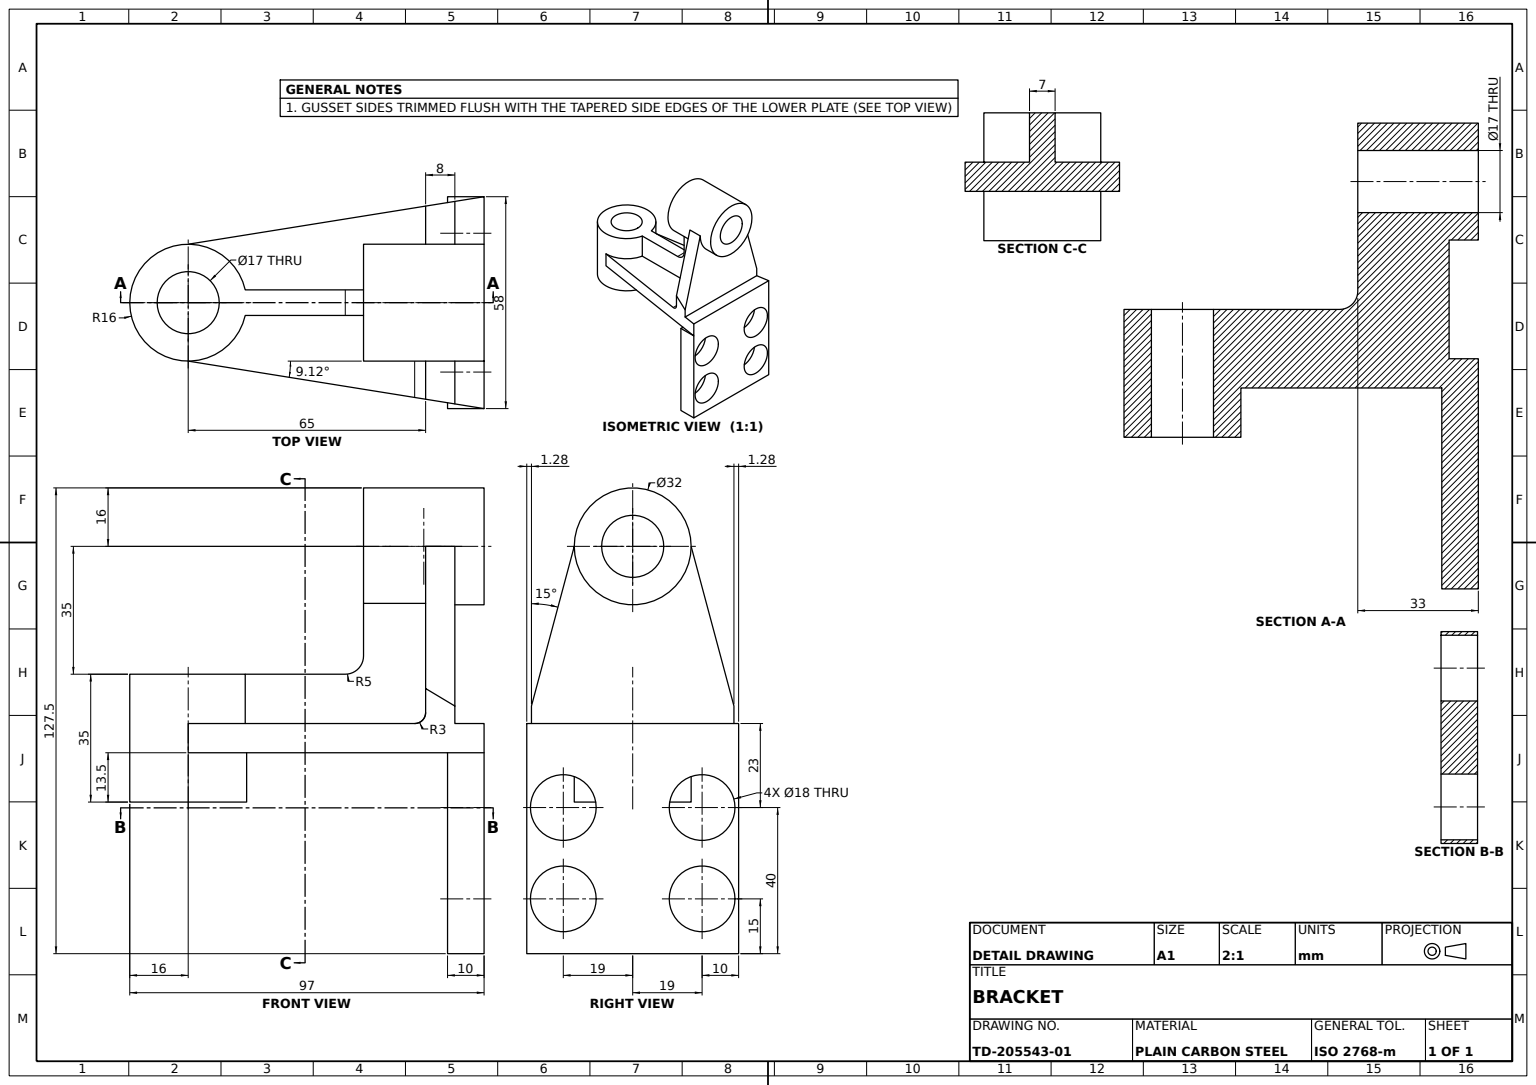
ISO-10303-21;
HEADER;
FILE_DESCRIPTION((''),'2;1');
FILE_NAME('','',(''),(''),'','','');
FILE_SCHEMA(('AUTOMOTIVE_DESIGN'));
ENDSEC;
DATA;
#1=APPLICATION_CONTEXT('');
#2=PRODUCT_CONTEXT('',#1,'mechanical');
#3=PRODUCT('','','',(#2));
#4=PRODUCT_DEFINITION_FORMATION('','',#3);
#5=PRODUCT_DEFINITION_CONTEXT('',#1,'design');
#6=PRODUCT_DEFINITION('','',#4,#5);
#7=PRODUCT_DEFINITION_SHAPE('','',#6);
#8=(LENGTH_UNIT()NAMED_UNIT(*)SI_UNIT(.MILLI.,.METRE.));
#9=(NAMED_UNIT(*)PLANE_ANGLE_UNIT()SI_UNIT($,.RADIAN.));
#10=(NAMED_UNIT(*)SI_UNIT($,.STERADIAN.)SOLID_ANGLE_UNIT());
#11=UNCERTAINTY_MEASURE_WITH_UNIT(LENGTH_MEASURE(1.E-05),#8,'distance_accuracy_value','');
#12=(GEOMETRIC_REPRESENTATION_CONTEXT(3)GLOBAL_UNCERTAINTY_ASSIGNED_CONTEXT((#11))GLOBAL_UNIT_ASSIGNED_CONTEXT((#8,#9,#10))REPRESENTATION_CONTEXT('',''));
#13=CARTESIAN_POINT('',(26.432099,13.580247,-65.));
#14=VERTEX_POINT('',#13);
#15=CARTESIAN_POINT('',(26.432099,7.,-65.));
#16=VERTEX_POINT('',#15);
#17=CARTESIAN_POINT('',(26.432099,52.5,-65.));
#18=DIRECTION('',(0.,-1.,0.));
#19=VECTOR('',#18,1000.);
#20=LINE('',#17,#19);
#21=EDGE_CURVE('',#14,#16,#20,.T.);
#22=ORIENTED_EDGE('',*,*,#21,.F.);
#23=CARTESIAN_POINT('',(16.,52.5,-65.));
#24=VERTEX_POINT('',#23);
#25=DIRECTION('',(-0.258901995,0.965903596,0.));
#26=VECTOR('',#25,1000.);
#27=LINE('',#23,#26);
#28=EDGE_CURVE('',#14,#24,#27,.T.);
#29=ORIENTED_EDGE('',*,*,#28,.T.);
#30=CARTESIAN_POINT('',(3.5,36.887505,-65.));
#31=VERTEX_POINT('',#30);
#32=CARTESIAN_POINT('',(0.,52.5,-65.));
#33=DIRECTION('',(0.,0.,-1.));
#34=DIRECTION('',(1.,0.,0.));
#35=AXIS2_PLACEMENT_3D('',#32,#33,#34);
#36=CIRCLE('',#35,16.);
#37=EDGE_CURVE('',#24,#31,#36,.T.);
#38=ORIENTED_EDGE('',*,*,#37,.T.);
#39=CARTESIAN_POINT('',(3.5,7.,-65.));
#40=VERTEX_POINT('',#39);
#41=CARTESIAN_POINT('',(3.5,4.,-65.));
#42=DIRECTION('',(0.,1.,0.));
#43=VECTOR('',#42,1000.);
#44=LINE('',#41,#43);
#45=EDGE_CURVE('',#40,#31,#44,.T.);
#46=ORIENTED_EDGE('',*,*,#45,.F.);
#47=VECTOR('',#34,1000.);
#48=LINE('',#15,#47);
#49=EDGE_CURVE('',#40,#16,#48,.T.);
#50=ORIENTED_EDGE('',*,*,#49,.T.);
#51=EDGE_LOOP('',(#22,#29,#38,#46,#50));
#52=FACE_OUTER_BOUND('',#51,.T.);
#53=DIRECTION('',(0.,0.,1.));
#54=AXIS2_PLACEMENT_3D('',#32,#53,#34);
#55=PLANE('',#54);
#56=ADVANCED_FACE('',(#52),#55,.T.);
#57=CARTESIAN_POINT('',(28.,-44.,-71.));
#58=VERTEX_POINT('',#57);
#59=CARTESIAN_POINT('',(10.,-44.,-71.));
#60=VERTEX_POINT('',#59);
#61=CARTESIAN_POINT('',(19.,-44.,-71.));
#62=AXIS2_PLACEMENT_3D('',#61,#53,#34);
#63=CIRCLE('',#62,9.);
#64=EDGE_CURVE('',#58,#60,#63,.T.);
#65=ORIENTED_EDGE('',*,*,#64,.T.);
#66=CARTESIAN_POINT('',(10.,-44.,-81.));
#67=VERTEX_POINT('',#66);
#68=CARTESIAN_POINT('',(10.,-44.,-126.));
#69=VECTOR('',#53,1000.);
#70=LINE('',#68,#69);
#71=EDGE_CURVE('',#67,#60,#70,.T.);
#72=ORIENTED_EDGE('',*,*,#71,.F.);
#73=CARTESIAN_POINT('',(28.,-44.,-81.));
#74=VERTEX_POINT('',#73);
#75=CARTESIAN_POINT('',(19.,-44.,-81.));
#76=AXIS2_PLACEMENT_3D('',#75,#53,#34);
#77=CIRCLE('',#76,9.);
#78=EDGE_CURVE('',#74,#67,#77,.T.);
#79=ORIENTED_EDGE('',*,*,#78,.F.);
#80=CARTESIAN_POINT('',(28.,-44.,-126.));
#81=LINE('',#80,#69);
#82=EDGE_CURVE('',#74,#58,#81,.T.);
#83=ORIENTED_EDGE('',*,*,#82,.T.);
#84=EDGE_LOOP('',(#65,#72,#79,#83));
#85=FACE_OUTER_BOUND('',#84,.T.);
#86=CARTESIAN_POINT('',(19.,-44.,-126.));
#87=AXIS2_PLACEMENT_3D('',#86,#53,#34);
#88=CYLINDRICAL_SURFACE('',#87,9.);
#89=ADVANCED_FACE('',(#85),#88,.F.);
#90=CARTESIAN_POINT('',(-28.,-44.,-81.));
#91=VERTEX_POINT('',#90);
#92=CARTESIAN_POINT('',(-28.,-44.,-71.));
#93=VERTEX_POINT('',#92);
#94=CARTESIAN_POINT('',(-28.,-44.,-126.));
#95=LINE('',#94,#69);
#96=EDGE_CURVE('',#91,#93,#95,.T.);
#97=ORIENTED_EDGE('',*,*,#96,.F.);
#98=CARTESIAN_POINT('',(-10.,-44.,-81.));
#99=VERTEX_POINT('',#98);
#100=CARTESIAN_POINT('',(-19.,-44.,-81.));
#101=AXIS2_PLACEMENT_3D('',#100,#53,#34);
#102=CIRCLE('',#101,9.);
#103=EDGE_CURVE('',#99,#91,#102,.T.);
#104=ORIENTED_EDGE('',*,*,#103,.F.);
#105=CARTESIAN_POINT('',(-10.,-44.,-71.));
#106=VERTEX_POINT('',#105);
#107=CARTESIAN_POINT('',(-10.,-44.,-126.));
#108=LINE('',#107,#69);
#109=EDGE_CURVE('',#99,#106,#108,.T.);
#110=ORIENTED_EDGE('',*,*,#109,.T.);
#111=CARTESIAN_POINT('',(-19.,-44.,-71.));
#112=DIRECTION('',(-1.,0.,0.));
#113=AXIS2_PLACEMENT_3D('',#111,#53,#112);
#114=CIRCLE('',#113,9.);
#115=EDGE_CURVE('',#106,#93,#114,.T.);
#116=ORIENTED_EDGE('',*,*,#115,.T.);
#117=EDGE_LOOP('',(#97,#104,#110,#116));
#118=FACE_OUTER_BOUND('',#117,.T.);
#119=CARTESIAN_POINT('',(-19.,-44.,-126.));
#120=AXIS2_PLACEMENT_3D('',#119,#53,#34);
#121=CYLINDRICAL_SURFACE('',#120,9.);
#122=ADVANCED_FACE('',(#118),#121,.F.);
#123=CARTESIAN_POINT('',(-16.,52.5,-73.));
#124=VERTEX_POINT('',#123);
#125=CARTESIAN_POINT('',(-27.716049,8.790123,-73.));
#126=VERTEX_POINT('',#125);
#127=DIRECTION('',(-0.258901995,-0.965903596,0.));
#128=VECTOR('',#127,1000.);
#129=LINE('',#123,#128);
#130=EDGE_CURVE('',#124,#126,#129,.T.);
#131=ORIENTED_EDGE('',*,*,#130,.T.);
#132=CARTESIAN_POINT('',(-26.432099,13.580247,-65.));
#133=VERTEX_POINT('',#132);
#134=CARTESIAN_POINT('',(-24.463652,20.924069,-52.73506));
#135=DIRECTION('',(-0.136410131,-0.50891472,-0.849940047));
#136=VECTOR('',#135,1000.);
#137=LINE('',#134,#136);
#138=EDGE_CURVE('',#133,#126,#137,.T.);
#139=ORIENTED_EDGE('',*,*,#138,.F.);
#140=CARTESIAN_POINT('',(-16.,52.5,-65.));
#141=VERTEX_POINT('',#140);
#142=LINE('',#140,#128);
#143=EDGE_CURVE('',#141,#133,#142,.T.);
#144=ORIENTED_EDGE('',*,*,#143,.F.);
#145=LINE('',#123,#69);
#146=EDGE_CURVE('',#124,#141,#145,.T.);
#147=ORIENTED_EDGE('',*,*,#146,.F.);
#148=EDGE_LOOP('',(#131,#139,#144,#147));
#149=FACE_OUTER_BOUND('',#148,.T.);
#150=DIRECTION('',(-0.965903596,0.258901995,0.));
#151=AXIS2_PLACEMENT_3D('',#123,#150,#127);
#152=PLANE('',#151);
#153=ADVANCED_FACE('',(#149),#152,.T.);
#154=CARTESIAN_POINT('',(-29.,-4.,-71.));
#155=VERTEX_POINT('',#154);
#156=CARTESIAN_POINT('',(-29.,-4.,-81.));
#157=VERTEX_POINT('',#156);
#158=VECTOR('',#33,1000.);
#159=LINE('',#154,#158);
#160=EDGE_CURVE('',#155,#157,#159,.T.);
#161=ORIENTED_EDGE('',*,*,#160,.F.);
#162=CARTESIAN_POINT('',(-27.395062,-4.,-71.));
#163=VERTEX_POINT('',#162);
#164=CARTESIAN_POINT('',(29.,-4.,-71.));
#165=VECTOR('',#112,1000.);
#166=LINE('',#164,#165);
#167=EDGE_CURVE('',#163,#155,#166,.T.);
#168=ORIENTED_EDGE('',*,*,#167,.F.);
#169=DIRECTION('',(0.1584659,0.,0.987364451));
#170=VECTOR('',#169,1000.);
#171=LINE('',#156,#170);
#172=EDGE_CURVE('',#157,#163,#171,.T.);
#173=ORIENTED_EDGE('',*,*,#172,.F.);
#174=EDGE_LOOP('',(#161,#168,#173));
#175=FACE_OUTER_BOUND('',#174,.T.);
#176=CARTESIAN_POINT('',(0.,-4.,0.));
#177=AXIS2_PLACEMENT_3D('',#176,#18,#33);
#178=PLANE('',#177);
#179=ADVANCED_FACE('',(#175),#178,.F.);
#180=CARTESIAN_POINT('',(0.,-17.5,8.5));
#181=VERTEX_POINT('',#180);
#182=CARTESIAN_POINT('',(0.,17.5,8.5));
#183=VERTEX_POINT('',#182);
#184=CARTESIAN_POINT('',(0.,-39.5,8.5));
#185=LINE('',#184,#43);
#186=EDGE_CURVE('',#181,#183,#185,.T.);
#187=ORIENTED_EDGE('',*,*,#186,.T.);
#188=CARTESIAN_POINT('',(0.,17.5,-8.5));
#189=VERTEX_POINT('',#188);
#190=CARTESIAN_POINT('',(0.,17.5,0.));
#191=AXIS2_PLACEMENT_3D('',#190,#42,#53);
#192=CIRCLE('',#191,8.5);
#193=EDGE_CURVE('',#183,#189,#192,.T.);
#194=ORIENTED_EDGE('',*,*,#193,.T.);
#195=CARTESIAN_POINT('',(0.,-17.5,-8.5));
#196=VERTEX_POINT('',#195);
#197=CARTESIAN_POINT('',(0.,-39.5,-8.5));
#198=LINE('',#197,#43);
#199=EDGE_CURVE('',#196,#189,#198,.T.);
#200=ORIENTED_EDGE('',*,*,#199,.F.);
#201=CARTESIAN_POINT('',(0.,-17.5,0.));
#202=AXIS2_PLACEMENT_3D('',#201,#42,#53);
#203=CIRCLE('',#202,8.5);
#204=EDGE_CURVE('',#181,#196,#203,.T.);
#205=ORIENTED_EDGE('',*,*,#204,.F.);
#206=EDGE_LOOP('',(#187,#194,#200,#205));
#207=FACE_OUTER_BOUND('',#206,.T.);
#208=CARTESIAN_POINT('',(0.,-39.5,0.));
#209=AXIS2_PLACEMENT_3D('',#208,#42,#53);
#210=CYLINDRICAL_SURFACE('',#209,8.5);
#211=ADVANCED_FACE('',(#207),#210,.F.);
#212=VERTEX_POINT('',#164);
#213=CARTESIAN_POINT('',(27.395062,-4.,-71.));
#214=VERTEX_POINT('',#213);
#215=EDGE_CURVE('',#212,#214,#166,.T.);
#216=ORIENTED_EDGE('',*,*,#215,.F.);
#217=CARTESIAN_POINT('',(29.,-4.,-81.));
#218=VERTEX_POINT('',#217);
#219=LINE('',#217,#69);
#220=EDGE_CURVE('',#218,#212,#219,.T.);
#221=ORIENTED_EDGE('',*,*,#220,.F.);
#222=DIRECTION('',(0.1584659,0.,-0.987364451));
#223=VECTOR('',#222,1000.);
#224=LINE('',#217,#223);
#225=EDGE_CURVE('',#214,#218,#224,.T.);
#226=ORIENTED_EDGE('',*,*,#225,.F.);
#227=EDGE_LOOP('',(#216,#221,#226));
#228=FACE_OUTER_BOUND('',#227,.T.);
#229=ADVANCED_FACE('',(#228),#178,.F.);
#230=ORIENTED_EDGE('',*,*,#199,.T.);
#231=EDGE_CURVE('',#189,#183,#192,.T.);
#232=ORIENTED_EDGE('',*,*,#231,.T.);
#233=ORIENTED_EDGE('',*,*,#186,.F.);
#234=EDGE_CURVE('',#196,#181,#203,.T.);
#235=ORIENTED_EDGE('',*,*,#234,.F.);
#236=EDGE_LOOP('',(#230,#232,#233,#235));
#237=FACE_OUTER_BOUND('',#236,.T.);
#238=ADVANCED_FACE('',(#237),#210,.F.);
#239=CARTESIAN_POINT('',(-29.,4.,-81.));
#240=VERTEX_POINT('',#239);
#241=CARTESIAN_POINT('',(-27.716049,4.,-73.));
#242=VERTEX_POINT('',#241);
#243=LINE('',#239,#170);
#244=EDGE_CURVE('',#240,#242,#243,.T.);
#245=ORIENTED_EDGE('',*,*,#244,.T.);
#246=CARTESIAN_POINT('',(27.716049,4.,-73.));
#247=VERTEX_POINT('',#246);
#248=CARTESIAN_POINT('',(0.,4.,-73.));
#249=LINE('',#248,#47);
#250=EDGE_CURVE('',#242,#247,#249,.T.);
#251=ORIENTED_EDGE('',*,*,#250,.T.);
#252=CARTESIAN_POINT('',(29.,4.,-81.));
#253=VERTEX_POINT('',#252);
#254=LINE('',#252,#223);
#255=EDGE_CURVE('',#247,#253,#254,.T.);
#256=ORIENTED_EDGE('',*,*,#255,.T.);
#257=CARTESIAN_POINT('',(0.,4.,-81.));
#258=LINE('',#257,#165);
#259=EDGE_CURVE('',#253,#240,#258,.T.);
#260=ORIENTED_EDGE('',*,*,#259,.T.);
#261=EDGE_LOOP('',(#245,#251,#256,#260));
#262=FACE_OUTER_BOUND('',#261,.T.);
#263=CARTESIAN_POINT('',(0.,4.,0.));
#264=AXIS2_PLACEMENT_3D('',#263,#42,#53);
#265=PLANE('',#264);
#266=ADVANCED_FACE('',(#262),#265,.T.);
#267=CARTESIAN_POINT('',(0.,-17.5,16.));
#268=VERTEX_POINT('',#267);
#269=CARTESIAN_POINT('',(0.,-17.5,-16.));
#270=VERTEX_POINT('',#269);
#271=CIRCLE('',#202,16.);
#272=EDGE_CURVE('',#268,#270,#271,.T.);
#273=ORIENTED_EDGE('',*,*,#272,.F.);
#274=EDGE_CURVE('',#270,#268,#271,.T.);
#275=ORIENTED_EDGE('',*,*,#274,.F.);
#276=EDGE_LOOP('',(#273,#275));
#277=FACE_OUTER_BOUND('',#276,.T.);
#278=ORIENTED_EDGE('',*,*,#234,.T.);
#279=ORIENTED_EDGE('',*,*,#204,.T.);
#280=EDGE_LOOP('',(#278,#279));
#281=FACE_BOUND('',#280,.T.);
#282=PLANE('',#202);
#283=ADVANCED_FACE('',(#277,#281),#282,.F.);
#284=CARTESIAN_POINT('',(-26.432099,4.,-65.));
#285=VERTEX_POINT('',#284);
#286=CARTESIAN_POINT('',(-16.,4.,0.));
#287=VERTEX_POINT('',#286);
#288=EDGE_CURVE('',#285,#287,#243,.T.);
#289=ORIENTED_EDGE('',*,*,#288,.F.);
#290=CARTESIAN_POINT('',(-26.432099,52.5,-65.));
#291=LINE('',#290,#43);
#292=EDGE_CURVE('',#285,#133,#291,.T.);
#293=ORIENTED_EDGE('',*,*,#292,.T.);
#294=ORIENTED_EDGE('',*,*,#138,.T.);
#295=CARTESIAN_POINT('',(-27.716049,34.,-73.));
#296=LINE('',#295,#19);
#297=EDGE_CURVE('',#126,#242,#296,.T.);
#298=ORIENTED_EDGE('',*,*,#297,.T.);
#299=ORIENTED_EDGE('',*,*,#244,.F.);
#300=LINE('',#239,#19);
#301=EDGE_CURVE('',#240,#157,#300,.T.);
#302=ORIENTED_EDGE('',*,*,#301,.T.);
#303=ORIENTED_EDGE('',*,*,#172,.T.);
#304=CARTESIAN_POINT('',(-16.,-4.,0.));
#305=VERTEX_POINT('',#304);
#306=EDGE_CURVE('',#163,#305,#171,.T.);
#307=ORIENTED_EDGE('',*,*,#306,.T.);
#308=LINE('',#286,#19);
#309=EDGE_CURVE('',#287,#305,#308,.T.);
#310=ORIENTED_EDGE('',*,*,#309,.F.);
#311=EDGE_LOOP('',(#289,#293,#294,#298,#299,#302,#303,#307,#310));
#312=FACE_OUTER_BOUND('',#311,.T.);
#313=DIRECTION('',(0.987364451,0.,-0.1584659));
#314=DIRECTION('',(-0.1584659,0.,-0.987364451));
#315=AXIS2_PLACEMENT_3D('',#239,#313,#314);
#316=PLANE('',#315);
#317=ADVANCED_FACE('',(#312),#316,.F.);
#318=CARTESIAN_POINT('',(10.,-19.,-81.));
#319=VERTEX_POINT('',#318);
#320=CARTESIAN_POINT('',(10.,-19.,-71.));
#321=VERTEX_POINT('',#320);
#322=CARTESIAN_POINT('',(10.,-19.,-126.));
#323=LINE('',#322,#69);
#324=EDGE_CURVE('',#319,#321,#323,.T.);
#325=ORIENTED_EDGE('',*,*,#324,.F.);
#326=CARTESIAN_POINT('',(28.,-19.,-81.));
#327=VERTEX_POINT('',#326);
#328=CARTESIAN_POINT('',(19.,-19.,-81.));
#329=AXIS2_PLACEMENT_3D('',#328,#53,#34);
#330=CIRCLE('',#329,9.);
#331=EDGE_CURVE('',#327,#319,#330,.T.);
#332=ORIENTED_EDGE('',*,*,#331,.F.);
#333=CARTESIAN_POINT('',(28.,-19.,-71.));
#334=VERTEX_POINT('',#333);
#335=CARTESIAN_POINT('',(28.,-19.,-126.));
#336=LINE('',#335,#69);
#337=EDGE_CURVE('',#327,#334,#336,.T.);
#338=ORIENTED_EDGE('',*,*,#337,.T.);
#339=CARTESIAN_POINT('',(19.,-19.,-71.));
#340=AXIS2_PLACEMENT_3D('',#339,#53,#112);
#341=CIRCLE('',#340,9.);
#342=EDGE_CURVE('',#334,#321,#341,.T.);
#343=ORIENTED_EDGE('',*,*,#342,.T.);
#344=EDGE_LOOP('',(#325,#332,#338,#343));
#345=FACE_OUTER_BOUND('',#344,.T.);
#346=CARTESIAN_POINT('',(19.,-19.,-126.));
#347=AXIS2_PLACEMENT_3D('',#346,#53,#34);
#348=CYLINDRICAL_SURFACE('',#347,9.);
#349=ADVANCED_FACE('',(#345),#348,.F.);
#350=ORIENTED_EDGE('',*,*,#324,.T.);
#351=EDGE_CURVE('',#321,#334,#341,.T.);
#352=ORIENTED_EDGE('',*,*,#351,.T.);
#353=ORIENTED_EDGE('',*,*,#337,.F.);
#354=EDGE_CURVE('',#319,#327,#330,.T.);
#355=ORIENTED_EDGE('',*,*,#354,.F.);
#356=EDGE_LOOP('',(#350,#352,#353,#355));
#357=FACE_OUTER_BOUND('',#356,.T.);
#358=ADVANCED_FACE('',(#357),#348,.F.);
#359=EDGE_CURVE('',#60,#58,#63,.T.);
#360=ORIENTED_EDGE('',*,*,#359,.T.);
#361=ORIENTED_EDGE('',*,*,#82,.F.);
#362=EDGE_CURVE('',#67,#74,#77,.T.);
#363=ORIENTED_EDGE('',*,*,#362,.F.);
#364=ORIENTED_EDGE('',*,*,#71,.T.);
#365=EDGE_LOOP('',(#360,#361,#363,#364));
#366=FACE_OUTER_BOUND('',#365,.T.);
#367=ADVANCED_FACE('',(#366),#88,.F.);
#368=CARTESIAN_POINT('',(8.5,52.5,-81.));
#369=VERTEX_POINT('',#368);
#370=CARTESIAN_POINT('',(8.5,52.5,-48.));
#371=VERTEX_POINT('',#370);
#372=CARTESIAN_POINT('',(8.5,52.5,-86.));
#373=LINE('',#372,#69);
#374=EDGE_CURVE('',#369,#371,#373,.T.);
#375=ORIENTED_EDGE('',*,*,#374,.T.);
#376=CARTESIAN_POINT('',(-8.5,52.5,-48.));
#377=VERTEX_POINT('',#376);
#378=CARTESIAN_POINT('',(0.,52.5,-48.));
#379=AXIS2_PLACEMENT_3D('',#378,#53,#34);
#380=CIRCLE('',#379,8.5);
#381=EDGE_CURVE('',#371,#377,#380,.T.);
#382=ORIENTED_EDGE('',*,*,#381,.T.);
#383=CARTESIAN_POINT('',(-8.5,52.5,-81.));
#384=VERTEX_POINT('',#383);
#385=CARTESIAN_POINT('',(-8.5,52.5,-86.));
#386=LINE('',#385,#69);
#387=EDGE_CURVE('',#384,#377,#386,.T.);
#388=ORIENTED_EDGE('',*,*,#387,.F.);
#389=CARTESIAN_POINT('',(0.,52.5,-81.));
#390=AXIS2_PLACEMENT_3D('',#389,#53,#34);
#391=CIRCLE('',#390,8.5);
#392=EDGE_CURVE('',#369,#384,#391,.T.);
#393=ORIENTED_EDGE('',*,*,#392,.F.);
#394=EDGE_LOOP('',(#375,#382,#388,#393));
#395=FACE_OUTER_BOUND('',#394,.T.);
#396=CARTESIAN_POINT('',(0.,52.5,-86.));
#397=AXIS2_PLACEMENT_3D('',#396,#53,#34);
#398=CYLINDRICAL_SURFACE('',#397,8.5);
#399=ADVANCED_FACE('',(#395),#398,.F.);
#400=CARTESIAN_POINT('',(3.5,22.5,-48.));
#401=VERTEX_POINT('',#400);
#402=CARTESIAN_POINT('',(3.5,17.5,-43.));
#403=VERTEX_POINT('',#402);
#404=CARTESIAN_POINT('',(3.5,22.5,-43.));
#405=AXIS2_PLACEMENT_3D('',#404,#112,#33);
#406=CIRCLE('',#405,5.);
#407=EDGE_CURVE('',#401,#403,#406,.T.);
#408=ORIENTED_EDGE('',*,*,#407,.F.);
#409=CARTESIAN_POINT('',(-3.5,22.5,-48.));
#410=VERTEX_POINT('',#409);
#411=LINE('',#400,#47);
#412=EDGE_CURVE('',#410,#401,#411,.T.);
#413=ORIENTED_EDGE('',*,*,#412,.F.);
#414=CARTESIAN_POINT('',(-3.5,17.5,-43.));
#415=VERTEX_POINT('',#414);
#416=CARTESIAN_POINT('',(-3.5,22.5,-43.));
#417=AXIS2_PLACEMENT_3D('',#416,#34,#33);
#418=CIRCLE('',#417,5.);
#419=EDGE_CURVE('',#415,#410,#418,.T.);
#420=ORIENTED_EDGE('',*,*,#419,.F.);
#421=LINE('',#414,#165);
#422=EDGE_CURVE('',#403,#415,#421,.T.);
#423=ORIENTED_EDGE('',*,*,#422,.F.);
#424=EDGE_LOOP('',(#408,#413,#420,#423));
#425=FACE_OUTER_BOUND('',#424,.T.);
#426=CARTESIAN_POINT('',(0.,22.5,-43.));
#427=AXIS2_PLACEMENT_3D('',#426,#34,#33);
#428=CYLINDRICAL_SURFACE('',#427,5.);
#429=ADVANCED_FACE('',(#425),#428,.F.);
#430=ORIENTED_EDGE('',*,*,#193,.F.);
#431=ORIENTED_EDGE('',*,*,#231,.F.);
#432=EDGE_LOOP('',(#430,#431));
#433=FACE_BOUND('',#432,.T.);
#434=CARTESIAN_POINT('',(-3.5,17.5,-15.612495));
#435=VERTEX_POINT('',#434);
#436=CARTESIAN_POINT('',(-3.5,17.5,-48.));
#437=LINE('',#436,#69);
#438=EDGE_CURVE('',#415,#435,#437,.T.);
#439=ORIENTED_EDGE('',*,*,#438,.T.);
#440=CARTESIAN_POINT('',(0.,17.5,16.));
#441=VERTEX_POINT('',#440);
#442=CIRCLE('',#191,16.);
#443=EDGE_CURVE('',#435,#441,#442,.T.);
#444=ORIENTED_EDGE('',*,*,#443,.T.);
#445=CARTESIAN_POINT('',(3.5,17.5,-15.612495));
#446=VERTEX_POINT('',#445);
#447=EDGE_CURVE('',#441,#446,#442,.T.);
#448=ORIENTED_EDGE('',*,*,#447,.T.);
#449=CARTESIAN_POINT('',(3.5,17.5,-48.));
#450=LINE('',#449,#69);
#451=EDGE_CURVE('',#403,#446,#450,.T.);
#452=ORIENTED_EDGE('',*,*,#451,.F.);
#453=ORIENTED_EDGE('',*,*,#422,.T.);
#454=EDGE_LOOP('',(#439,#444,#448,#452,#453));
#455=FACE_OUTER_BOUND('',#454,.T.);
#456=PLANE('',#191);
#457=ADVANCED_FACE('',(#433,#455),#456,.T.);
#458=CARTESIAN_POINT('',(-3.5,36.887505,-65.));
#459=VERTEX_POINT('',#458);
#460=EDGE_CURVE('',#459,#141,#36,.T.);
#461=ORIENTED_EDGE('',*,*,#460,.F.);
#462=CARTESIAN_POINT('',(-3.5,36.887505,-48.));
#463=VERTEX_POINT('',#462);
#464=CARTESIAN_POINT('',(-3.5,36.887505,-81.));
#465=LINE('',#464,#69);
#466=EDGE_CURVE('',#459,#463,#465,.T.);
#467=ORIENTED_EDGE('',*,*,#466,.T.);
#468=CARTESIAN_POINT('',(-16.,52.5,-48.));
#469=VERTEX_POINT('',#468);
#470=CIRCLE('',#379,16.);
#471=EDGE_CURVE('',#469,#463,#470,.T.);
#472=ORIENTED_EDGE('',*,*,#471,.F.);
#473=CARTESIAN_POINT('',(-16.,52.5,-81.));
#474=LINE('',#473,#69);
#475=EDGE_CURVE('',#141,#469,#474,.T.);
#476=ORIENTED_EDGE('',*,*,#475,.F.);
#477=EDGE_LOOP('',(#461,#467,#472,#476));
#478=FACE_OUTER_BOUND('',#477,.T.);
#479=CYLINDRICAL_SURFACE('',#390,16.);
#480=ADVANCED_FACE('',(#478),#479,.T.);
#481=ORIENTED_EDGE('',*,*,#407,.T.);
#482=ORIENTED_EDGE('',*,*,#451,.T.);
#483=CARTESIAN_POINT('',(3.5,4.,-15.612495));
#484=VERTEX_POINT('',#483);
#485=CARTESIAN_POINT('',(3.5,-17.5,-15.612495));
#486=LINE('',#485,#19);
#487=EDGE_CURVE('',#446,#484,#486,.T.);
#488=ORIENTED_EDGE('',*,*,#487,.T.);
#489=CARTESIAN_POINT('',(3.5,4.,-62.));
#490=VERTEX_POINT('',#489);
#491=CARTESIAN_POINT('',(3.5,4.,-11.269108));
#492=LINE('',#491,#158);
#493=EDGE_CURVE('',#484,#490,#492,.T.);
#494=ORIENTED_EDGE('',*,*,#493,.T.);
#495=CARTESIAN_POINT('',(3.5,7.,-62.));
#496=AXIS2_PLACEMENT_3D('',#495,#34,#33);
#497=CIRCLE('',#496,3.);
#498=EDGE_CURVE('',#490,#40,#497,.T.);
#499=ORIENTED_EDGE('',*,*,#498,.T.);
#500=ORIENTED_EDGE('',*,*,#45,.T.);
#501=CARTESIAN_POINT('',(3.5,36.887505,-48.));
#502=VERTEX_POINT('',#501);
#503=CARTESIAN_POINT('',(3.5,36.887505,-81.));
#504=LINE('',#503,#69);
#505=EDGE_CURVE('',#31,#502,#504,.T.);
#506=ORIENTED_EDGE('',*,*,#505,.T.);
#507=CARTESIAN_POINT('',(3.5,40.002332,-48.));
#508=LINE('',#507,#19);
#509=EDGE_CURVE('',#502,#401,#508,.T.);
#510=ORIENTED_EDGE('',*,*,#509,.T.);
#511=EDGE_LOOP('',(#481,#482,#488,#494,#499,#500,#506,#510));
#512=FACE_OUTER_BOUND('',#511,.T.);
#513=CARTESIAN_POINT('',(3.5,0.,0.));
#514=AXIS2_PLACEMENT_3D('',#513,#34,#33);
#515=PLANE('',#514);
#516=ADVANCED_FACE('',(#512),#515,.T.);
#517=ORIENTED_EDGE('',*,*,#225,.T.);
#518=LINE('',#252,#19);
#519=EDGE_CURVE('',#253,#218,#518,.T.);
#520=ORIENTED_EDGE('',*,*,#519,.F.);
#521=ORIENTED_EDGE('',*,*,#255,.F.);
#522=CARTESIAN_POINT('',(27.716049,8.790123,-73.));
#523=VERTEX_POINT('',#522);
#524=CARTESIAN_POINT('',(27.716049,34.,-73.));
#525=LINE('',#524,#19);
#526=EDGE_CURVE('',#523,#247,#525,.T.);
#527=ORIENTED_EDGE('',*,*,#526,.F.);
#528=CARTESIAN_POINT('',(24.463652,20.924069,-52.73506));
#529=DIRECTION('',(-0.136410131,0.50891472,0.849940047));
#530=VECTOR('',#529,1000.);
#531=LINE('',#528,#530);
#532=EDGE_CURVE('',#523,#14,#531,.T.);
#533=ORIENTED_EDGE('',*,*,#532,.T.);
#534=ORIENTED_EDGE('',*,*,#21,.T.);
#535=CARTESIAN_POINT('',(25.950617,4.,-62.));
#536=VERTEX_POINT('',#535);
#537=CARTESIAN_POINT('',(26.432099,5.242641,-65.));
#538=CARTESIAN_POINT('',(26.232663,4.,-63.757359));
#539=(BOUNDED_CURVE()B_SPLINE_CURVE(3,(#15,#537,#538,#535),.UNSPECIFIED.,.F.,.F.)B_SPLINE_CURVE_WITH_KNOTS((4,4),(3.141592654,4.71238898),.UNSPECIFIED.)CURVE()GEOMETRIC_REPRESENTATION_ITEM()RATIONAL_B_SPLINE_CURVE((1.,0.804737854,0.804737854,1.))REPRESENTATION_ITEM(''));
#540=EDGE_CURVE('',#16,#536,#539,.T.);
#541=ORIENTED_EDGE('',*,*,#540,.T.);
#542=CARTESIAN_POINT('',(16.,4.,0.));
#543=VERTEX_POINT('',#542);
#544=EDGE_CURVE('',#543,#536,#254,.T.);
#545=ORIENTED_EDGE('',*,*,#544,.F.);
#546=CARTESIAN_POINT('',(16.,-4.,0.));
#547=VERTEX_POINT('',#546);
#548=LINE('',#542,#19);
#549=EDGE_CURVE('',#543,#547,#548,.T.);
#550=ORIENTED_EDGE('',*,*,#549,.T.);
#551=EDGE_CURVE('',#547,#214,#224,.T.);
#552=ORIENTED_EDGE('',*,*,#551,.T.);
#553=EDGE_LOOP('',(#517,#520,#521,#527,#533,#534,#541,#545,#550,#552));
#554=FACE_OUTER_BOUND('',#553,.T.);
#555=DIRECTION('',(-0.987364451,0.,-0.1584659));
#556=DIRECTION('',(-0.1584659,0.,0.987364451));
#557=AXIS2_PLACEMENT_3D('',#252,#555,#556);
#558=PLANE('',#557);
#559=ADVANCED_FACE('',(#554),#558,.F.);
#560=ORIENTED_EDGE('',*,*,#392,.T.);
#561=EDGE_CURVE('',#384,#369,#391,.T.);
#562=ORIENTED_EDGE('',*,*,#561,.T.);
#563=EDGE_LOOP('',(#560,#562));
#564=FACE_BOUND('',#563,.T.);
#565=CARTESIAN_POINT('',(16.,52.5,-81.));
#566=VERTEX_POINT('',#565);
#567=VERTEX_POINT('',#473);
#568=CIRCLE('',#390,16.);
#569=EDGE_CURVE('',#566,#567,#568,.T.);
#570=ORIENTED_EDGE('',*,*,#569,.F.);
#571=EDGE_CURVE('',#567,#566,#568,.T.);
#572=ORIENTED_EDGE('',*,*,#571,.F.);
#573=EDGE_LOOP('',(#570,#572));
#574=FACE_OUTER_BOUND('',#573,.T.);
#575=CARTESIAN_POINT('',(0.,0.,-81.));
#576=AXIS2_PLACEMENT_3D('',#575,#53,#34);
#577=PLANE('',#576);
#578=ADVANCED_FACE('',(#564,#574),#577,.F.);
#579=ORIENTED_EDGE('',*,*,#37,.F.);
#580=CARTESIAN_POINT('',(16.,52.5,-48.));
#581=VERTEX_POINT('',#580);
#582=LINE('',#565,#69);
#583=EDGE_CURVE('',#24,#581,#582,.T.);
#584=ORIENTED_EDGE('',*,*,#583,.T.);
#585=EDGE_CURVE('',#502,#581,#470,.T.);
#586=ORIENTED_EDGE('',*,*,#585,.F.);
#587=ORIENTED_EDGE('',*,*,#505,.F.);
#588=EDGE_LOOP('',(#579,#584,#586,#587));
#589=FACE_OUTER_BOUND('',#588,.T.);
#590=ADVANCED_FACE('',(#589),#479,.T.);
#591=CARTESIAN_POINT('',(0.,-4.,-16.));
#592=VERTEX_POINT('',#591);
#593=AXIS2_PLACEMENT_3D('',#176,#18,#53);
#594=CIRCLE('',#593,16.);
#595=EDGE_CURVE('',#305,#592,#594,.T.);
#596=ORIENTED_EDGE('',*,*,#595,.T.);
#597=LINE('',#269,#43);
#598=EDGE_CURVE('',#270,#592,#597,.T.);
#599=ORIENTED_EDGE('',*,*,#598,.F.);
#600=ORIENTED_EDGE('',*,*,#274,.T.);
#601=LINE('',#267,#43);
#602=EDGE_CURVE('',#268,#441,#601,.T.);
#603=ORIENTED_EDGE('',*,*,#602,.T.);
#604=ORIENTED_EDGE('',*,*,#443,.F.);
#605=CARTESIAN_POINT('',(-3.5,4.,-15.612495));
#606=VERTEX_POINT('',#605);
#607=CARTESIAN_POINT('',(-3.5,-17.5,-15.612495));
#608=LINE('',#607,#19);
#609=EDGE_CURVE('',#435,#606,#608,.T.);
#610=ORIENTED_EDGE('',*,*,#609,.T.);
#611=AXIS2_PLACEMENT_3D('',#263,#18,#53);
#612=CIRCLE('',#611,16.);
#613=EDGE_CURVE('',#287,#606,#612,.T.);
#614=ORIENTED_EDGE('',*,*,#613,.F.);
#615=ORIENTED_EDGE('',*,*,#309,.T.);
#616=EDGE_LOOP('',(#596,#599,#600,#603,#604,#610,#614,#615));
#617=FACE_OUTER_BOUND('',#616,.T.);
#618=CYLINDRICAL_SURFACE('',#202,16.);
#619=ADVANCED_FACE('',(#617),#618,.T.);
#620=ORIENTED_EDGE('',*,*,#374,.F.);
#621=ORIENTED_EDGE('',*,*,#561,.F.);
#622=ORIENTED_EDGE('',*,*,#387,.T.);
#623=EDGE_CURVE('',#377,#371,#380,.T.);
#624=ORIENTED_EDGE('',*,*,#623,.T.);
#625=EDGE_LOOP('',(#620,#621,#622,#624));
#626=FACE_OUTER_BOUND('',#625,.T.);
#627=ADVANCED_FACE('',(#626),#398,.F.);
#628=ORIENTED_EDGE('',*,*,#419,.T.);
#629=CARTESIAN_POINT('',(-3.5,40.002332,-48.));
#630=LINE('',#629,#19);
#631=EDGE_CURVE('',#463,#410,#630,.T.);
#632=ORIENTED_EDGE('',*,*,#631,.F.);
#633=ORIENTED_EDGE('',*,*,#466,.F.);
#634=CARTESIAN_POINT('',(-3.5,4.,-65.));
#635=VERTEX_POINT('',#634);
#636=LINE('',#634,#43);
#637=EDGE_CURVE('',#635,#459,#636,.T.);
#638=ORIENTED_EDGE('',*,*,#637,.F.);
#639=CARTESIAN_POINT('',(-3.5,4.,-11.269108));
#640=LINE('',#639,#158);
#641=EDGE_CURVE('',#606,#635,#640,.T.);
#642=ORIENTED_EDGE('',*,*,#641,.F.);
#643=ORIENTED_EDGE('',*,*,#609,.F.);
#644=ORIENTED_EDGE('',*,*,#438,.F.);
#645=EDGE_LOOP('',(#628,#632,#633,#638,#642,#643,#644));
#646=FACE_OUTER_BOUND('',#645,.T.);
#647=CARTESIAN_POINT('',(-3.5,0.,0.));
#648=AXIS2_PLACEMENT_3D('',#647,#34,#33);
#649=PLANE('',#648);
#650=ADVANCED_FACE('',(#646),#649,.F.);
#651=ORIENTED_EDGE('',*,*,#447,.F.);
#652=ORIENTED_EDGE('',*,*,#602,.F.);
#653=ORIENTED_EDGE('',*,*,#272,.T.);
#654=ORIENTED_EDGE('',*,*,#598,.T.);
#655=EDGE_CURVE('',#592,#547,#594,.T.);
#656=ORIENTED_EDGE('',*,*,#655,.T.);
#657=ORIENTED_EDGE('',*,*,#549,.F.);
#658=EDGE_CURVE('',#484,#543,#612,.T.);
#659=ORIENTED_EDGE('',*,*,#658,.F.);
#660=ORIENTED_EDGE('',*,*,#487,.F.);
#661=EDGE_LOOP('',(#651,#652,#653,#654,#656,#657,#659,#660));
#662=FACE_OUTER_BOUND('',#661,.T.);
#663=ADVANCED_FACE('',(#662),#618,.T.);
#664=ORIENTED_EDGE('',*,*,#526,.T.);
#665=ORIENTED_EDGE('',*,*,#250,.F.);
#666=ORIENTED_EDGE('',*,*,#297,.F.);
#667=ORIENTED_EDGE('',*,*,#130,.F.);
#668=CARTESIAN_POINT('',(16.,52.5,-73.));
#669=VERTEX_POINT('',#668);
#670=CARTESIAN_POINT('',(0.,52.5,-73.));
#671=AXIS2_PLACEMENT_3D('',#670,#33,#34);
#672=CIRCLE('',#671,16.);
#673=EDGE_CURVE('',#669,#124,#672,.T.);
#674=ORIENTED_EDGE('',*,*,#673,.F.);
#675=LINE('',#668,#26);
#676=EDGE_CURVE('',#523,#669,#675,.T.);
#677=ORIENTED_EDGE('',*,*,#676,.F.);
#678=EDGE_LOOP('',(#664,#665,#666,#667,#674,#677));
#679=FACE_OUTER_BOUND('',#678,.T.);
#680=AXIS2_PLACEMENT_3D('',#670,#53,#34);
#681=PLANE('',#680);
#682=ADVANCED_FACE('',(#679),#681,.F.);
#683=ORIENTED_EDGE('',*,*,#623,.F.);
#684=ORIENTED_EDGE('',*,*,#381,.F.);
#685=EDGE_LOOP('',(#683,#684));
#686=FACE_BOUND('',#685,.T.);
#687=ORIENTED_EDGE('',*,*,#631,.T.);
#688=ORIENTED_EDGE('',*,*,#412,.T.);
#689=ORIENTED_EDGE('',*,*,#509,.F.);
#690=ORIENTED_EDGE('',*,*,#585,.T.);
#691=EDGE_CURVE('',#581,#469,#470,.T.);
#692=ORIENTED_EDGE('',*,*,#691,.T.);
#693=ORIENTED_EDGE('',*,*,#471,.T.);
#694=EDGE_LOOP('',(#687,#688,#689,#690,#692,#693));
#695=FACE_OUTER_BOUND('',#694,.T.);
#696=CARTESIAN_POINT('',(0.,0.,-48.));
#697=AXIS2_PLACEMENT_3D('',#696,#53,#34);
#698=PLANE('',#697);
#699=ADVANCED_FACE('',(#686,#695),#698,.T.);
#700=ORIENTED_EDGE('',*,*,#49,.F.);
#701=ORIENTED_EDGE('',*,*,#498,.F.);
#702=LINE('',#489,#165);
#703=EDGE_CURVE('',#536,#490,#702,.T.);
#704=ORIENTED_EDGE('',*,*,#703,.F.);
#705=ORIENTED_EDGE('',*,*,#540,.F.);
#706=EDGE_LOOP('',(#700,#701,#704,#705));
#707=FACE_OUTER_BOUND('',#706,.T.);
#708=CARTESIAN_POINT('',(0.,7.,-62.));
#709=AXIS2_PLACEMENT_3D('',#708,#112,#53);
#710=CYLINDRICAL_SURFACE('',#709,3.);
#711=ADVANCED_FACE('',(#707),#710,.F.);
#712=ORIENTED_EDGE('',*,*,#351,.F.);
#713=ORIENTED_EDGE('',*,*,#342,.F.);
#714=EDGE_LOOP('',(#712,#713));
#715=FACE_BOUND('',#714,.T.);
#716=ORIENTED_EDGE('',*,*,#64,.F.);
#717=ORIENTED_EDGE('',*,*,#359,.F.);
#718=EDGE_LOOP('',(#716,#717));
#719=FACE_BOUND('',#718,.T.);
#720=EDGE_CURVE('',#93,#106,#114,.T.);
#721=ORIENTED_EDGE('',*,*,#720,.F.);
#722=ORIENTED_EDGE('',*,*,#115,.F.);
#723=EDGE_LOOP('',(#721,#722));
#724=FACE_BOUND('',#723,.T.);
#725=ORIENTED_EDGE('',*,*,#215,.T.);
#726=CARTESIAN_POINT('',(0.,-4.,-71.));
#727=LINE('',#726,#165);
#728=EDGE_CURVE('',#214,#163,#727,.T.);
#729=ORIENTED_EDGE('',*,*,#728,.T.);
#730=ORIENTED_EDGE('',*,*,#167,.T.);
#731=CARTESIAN_POINT('',(-29.,-59.,-71.));
#732=VERTEX_POINT('',#731);
#733=LINE('',#731,#43);
#734=EDGE_CURVE('',#732,#155,#733,.T.);
#735=ORIENTED_EDGE('',*,*,#734,.F.);
#736=CARTESIAN_POINT('',(29.,-59.,-71.));
#737=VERTEX_POINT('',#736);
#738=LINE('',#736,#165);
#739=EDGE_CURVE('',#737,#732,#738,.T.);
#740=ORIENTED_EDGE('',*,*,#739,.F.);
#741=LINE('',#736,#43);
#742=EDGE_CURVE('',#737,#212,#741,.T.);
#743=ORIENTED_EDGE('',*,*,#742,.T.);
#744=EDGE_LOOP('',(#725,#729,#730,#735,#740,#743));
#745=FACE_OUTER_BOUND('',#744,.T.);
#746=CARTESIAN_POINT('',(-28.,-19.,-71.));
#747=VERTEX_POINT('',#746);
#748=CARTESIAN_POINT('',(-10.,-19.,-71.));
#749=VERTEX_POINT('',#748);
#750=CARTESIAN_POINT('',(-19.,-19.,-71.));
#751=AXIS2_PLACEMENT_3D('',#750,#53,#34);
#752=CIRCLE('',#751,9.);
#753=EDGE_CURVE('',#747,#749,#752,.T.);
#754=ORIENTED_EDGE('',*,*,#753,.F.);
#755=EDGE_CURVE('',#749,#747,#752,.T.);
#756=ORIENTED_EDGE('',*,*,#755,.F.);
#757=EDGE_LOOP('',(#754,#756));
#758=FACE_BOUND('',#757,.T.);
#759=AXIS2_PLACEMENT_3D('',#736,#33,#112);
#760=PLANE('',#759);
#761=ADVANCED_FACE('',(#715,#719,#724,#745,#758),#760,.F.);
#762=ORIENTED_EDGE('',*,*,#532,.F.);
#763=ORIENTED_EDGE('',*,*,#676,.T.);
#764=LINE('',#668,#69);
#765=EDGE_CURVE('',#669,#24,#764,.T.);
#766=ORIENTED_EDGE('',*,*,#765,.T.);
#767=ORIENTED_EDGE('',*,*,#28,.F.);
#768=EDGE_LOOP('',(#762,#763,#766,#767));
#769=FACE_OUTER_BOUND('',#768,.T.);
#770=DIRECTION('',(0.965903596,0.258901995,0.));
#771=AXIS2_PLACEMENT_3D('',#668,#770,#25);
#772=PLANE('',#771);
#773=ADVANCED_FACE('',(#769),#772,.T.);
#774=CARTESIAN_POINT('',(-10.,-19.,-81.));
#775=VERTEX_POINT('',#774);
#776=CARTESIAN_POINT('',(-10.,-19.,-126.));
#777=LINE('',#776,#69);
#778=EDGE_CURVE('',#775,#749,#777,.T.);
#779=ORIENTED_EDGE('',*,*,#778,.T.);
#780=ORIENTED_EDGE('',*,*,#755,.T.);
#781=CARTESIAN_POINT('',(-28.,-19.,-81.));
#782=VERTEX_POINT('',#781);
#783=CARTESIAN_POINT('',(-28.,-19.,-126.));
#784=LINE('',#783,#69);
#785=EDGE_CURVE('',#782,#747,#784,.T.);
#786=ORIENTED_EDGE('',*,*,#785,.F.);
#787=CARTESIAN_POINT('',(-19.,-19.,-81.));
#788=AXIS2_PLACEMENT_3D('',#787,#53,#34);
#789=CIRCLE('',#788,9.);
#790=EDGE_CURVE('',#775,#782,#789,.T.);
#791=ORIENTED_EDGE('',*,*,#790,.F.);
#792=EDGE_LOOP('',(#779,#780,#786,#791));
#793=FACE_OUTER_BOUND('',#792,.T.);
#794=CARTESIAN_POINT('',(-19.,-19.,-126.));
#795=AXIS2_PLACEMENT_3D('',#794,#53,#34);
#796=CYLINDRICAL_SURFACE('',#795,9.);
#797=ADVANCED_FACE('',(#793),#796,.F.);
#798=ORIENTED_EDGE('',*,*,#519,.T.);
#799=CARTESIAN_POINT('',(29.,-59.,-81.));
#800=VERTEX_POINT('',#799);
#801=LINE('',#799,#43);
#802=EDGE_CURVE('',#800,#218,#801,.T.);
#803=ORIENTED_EDGE('',*,*,#802,.F.);
#804=CARTESIAN_POINT('',(-29.,-59.,-81.));
#805=VERTEX_POINT('',#804);
#806=LINE('',#804,#47);
#807=EDGE_CURVE('',#805,#800,#806,.T.);
#808=ORIENTED_EDGE('',*,*,#807,.F.);
#809=LINE('',#804,#43);
#810=EDGE_CURVE('',#805,#157,#809,.T.);
#811=ORIENTED_EDGE('',*,*,#810,.T.);
#812=ORIENTED_EDGE('',*,*,#301,.F.);
#813=ORIENTED_EDGE('',*,*,#259,.F.);
#814=EDGE_LOOP('',(#798,#803,#808,#811,#812,#813));
#815=FACE_OUTER_BOUND('',#814,.T.);
#816=ORIENTED_EDGE('',*,*,#78,.T.);
#817=ORIENTED_EDGE('',*,*,#362,.T.);
#818=EDGE_LOOP('',(#816,#817));
#819=FACE_BOUND('',#818,.T.);
#820=ORIENTED_EDGE('',*,*,#103,.T.);
#821=EDGE_CURVE('',#91,#99,#102,.T.);
#822=ORIENTED_EDGE('',*,*,#821,.T.);
#823=EDGE_LOOP('',(#820,#822));
#824=FACE_BOUND('',#823,.T.);
#825=EDGE_CURVE('',#782,#775,#789,.T.);
#826=ORIENTED_EDGE('',*,*,#825,.T.);
#827=ORIENTED_EDGE('',*,*,#790,.T.);
#828=EDGE_LOOP('',(#826,#827));
#829=FACE_BOUND('',#828,.T.);
#830=ORIENTED_EDGE('',*,*,#331,.T.);
#831=ORIENTED_EDGE('',*,*,#354,.T.);
#832=EDGE_LOOP('',(#830,#831));
#833=FACE_BOUND('',#832,.T.);
#834=AXIS2_PLACEMENT_3D('',#257,#53,#34);
#835=PLANE('',#834);
#836=ADVANCED_FACE('',(#815,#819,#824,#829,#833),#835,.F.);
#837=ORIENTED_EDGE('',*,*,#802,.T.);
#838=ORIENTED_EDGE('',*,*,#220,.T.);
#839=ORIENTED_EDGE('',*,*,#742,.F.);
#840=LINE('',#799,#69);
#841=EDGE_CURVE('',#800,#737,#840,.T.);
#842=ORIENTED_EDGE('',*,*,#841,.F.);
#843=EDGE_LOOP('',(#837,#838,#839,#842));
#844=FACE_OUTER_BOUND('',#843,.T.);
#845=AXIS2_PLACEMENT_3D('',#799,#112,#53);
#846=PLANE('',#845);
#847=ADVANCED_FACE('',(#844),#846,.F.);
#848=ORIENTED_EDGE('',*,*,#703,.T.);
#849=ORIENTED_EDGE('',*,*,#493,.F.);
#850=ORIENTED_EDGE('',*,*,#658,.T.);
#851=ORIENTED_EDGE('',*,*,#544,.T.);
#852=EDGE_LOOP('',(#848,#849,#850,#851));
#853=FACE_OUTER_BOUND('',#852,.T.);
#854=ADVANCED_FACE('',(#853),#265,.T.);
#855=ORIENTED_EDGE('',*,*,#583,.F.);
#856=ORIENTED_EDGE('',*,*,#765,.F.);
#857=EDGE_CURVE('',#566,#669,#582,.T.);
#858=ORIENTED_EDGE('',*,*,#857,.F.);
#859=ORIENTED_EDGE('',*,*,#569,.T.);
#860=EDGE_CURVE('',#567,#124,#474,.T.);
#861=ORIENTED_EDGE('',*,*,#860,.T.);
#862=ORIENTED_EDGE('',*,*,#146,.T.);
#863=ORIENTED_EDGE('',*,*,#475,.T.);
#864=ORIENTED_EDGE('',*,*,#691,.F.);
#865=EDGE_LOOP('',(#855,#856,#858,#859,#861,#862,#863,#864));
#866=FACE_OUTER_BOUND('',#865,.T.);
#867=ADVANCED_FACE('',(#866),#479,.T.);
#868=ORIENTED_EDGE('',*,*,#739,.T.);
#869=LINE('',#731,#158);
#870=EDGE_CURVE('',#732,#805,#869,.T.);
#871=ORIENTED_EDGE('',*,*,#870,.T.);
#872=ORIENTED_EDGE('',*,*,#807,.T.);
#873=ORIENTED_EDGE('',*,*,#841,.T.);
#874=EDGE_LOOP('',(#868,#871,#872,#873));
#875=FACE_OUTER_BOUND('',#874,.T.);
#876=CARTESIAN_POINT('',(0.,-59.,0.));
#877=AXIS2_PLACEMENT_3D('',#876,#18,#33);
#878=PLANE('',#877);
#879=ADVANCED_FACE('',(#875),#878,.T.);
#880=ORIENTED_EDGE('',*,*,#595,.F.);
#881=ORIENTED_EDGE('',*,*,#306,.F.);
#882=ORIENTED_EDGE('',*,*,#728,.F.);
#883=ORIENTED_EDGE('',*,*,#551,.F.);
#884=ORIENTED_EDGE('',*,*,#655,.F.);
#885=EDGE_LOOP('',(#880,#881,#882,#883,#884));
#886=FACE_OUTER_BOUND('',#885,.T.);
#887=AXIS2_PLACEMENT_3D('',#176,#42,#53);
#888=PLANE('',#887);
#889=ADVANCED_FACE('',(#886),#888,.F.);
#890=ORIENTED_EDGE('',*,*,#857,.T.);
#891=ORIENTED_EDGE('',*,*,#673,.T.);
#892=ORIENTED_EDGE('',*,*,#860,.F.);
#893=ORIENTED_EDGE('',*,*,#571,.T.);
#894=EDGE_LOOP('',(#890,#891,#892,#893));
#895=FACE_OUTER_BOUND('',#894,.T.);
#896=ADVANCED_FACE('',(#895),#479,.T.);
#897=ORIENTED_EDGE('',*,*,#641,.T.);
#898=CARTESIAN_POINT('',(0.,4.,-65.));
#899=LINE('',#898,#47);
#900=EDGE_CURVE('',#285,#635,#899,.T.);
#901=ORIENTED_EDGE('',*,*,#900,.F.);
#902=ORIENTED_EDGE('',*,*,#288,.T.);
#903=ORIENTED_EDGE('',*,*,#613,.T.);
#904=EDGE_LOOP('',(#897,#901,#902,#903));
#905=FACE_OUTER_BOUND('',#904,.T.);
#906=ADVANCED_FACE('',(#905),#265,.T.);
#907=ORIENTED_EDGE('',*,*,#870,.F.);
#908=ORIENTED_EDGE('',*,*,#734,.T.);
#909=ORIENTED_EDGE('',*,*,#160,.T.);
#910=ORIENTED_EDGE('',*,*,#810,.F.);
#911=EDGE_LOOP('',(#907,#908,#909,#910));
#912=FACE_OUTER_BOUND('',#911,.T.);
#913=AXIS2_PLACEMENT_3D('',#731,#34,#33);
#914=PLANE('',#913);
#915=ADVANCED_FACE('',(#912),#914,.F.);
#916=ORIENTED_EDGE('',*,*,#637,.T.);
#917=ORIENTED_EDGE('',*,*,#460,.T.);
#918=ORIENTED_EDGE('',*,*,#143,.T.);
#919=ORIENTED_EDGE('',*,*,#292,.F.);
#920=ORIENTED_EDGE('',*,*,#900,.T.);
#921=EDGE_LOOP('',(#916,#917,#918,#919,#920));
#922=FACE_OUTER_BOUND('',#921,.T.);
#923=ADVANCED_FACE('',(#922),#55,.T.);
#924=ORIENTED_EDGE('',*,*,#785,.T.);
#925=ORIENTED_EDGE('',*,*,#753,.T.);
#926=ORIENTED_EDGE('',*,*,#778,.F.);
#927=ORIENTED_EDGE('',*,*,#825,.F.);
#928=EDGE_LOOP('',(#924,#925,#926,#927));
#929=FACE_OUTER_BOUND('',#928,.T.);
#930=ADVANCED_FACE('',(#929),#796,.F.);
#931=ORIENTED_EDGE('',*,*,#821,.F.);
#932=ORIENTED_EDGE('',*,*,#96,.T.);
#933=ORIENTED_EDGE('',*,*,#720,.T.);
#934=ORIENTED_EDGE('',*,*,#109,.F.);
#935=EDGE_LOOP('',(#931,#932,#933,#934));
#936=FACE_OUTER_BOUND('',#935,.T.);
#937=ADVANCED_FACE('',(#936),#121,.F.);
#938=CLOSED_SHELL('',(#56,#89,#122,#153,#179,#211,#229,#238,#266,#283,#317,#349,#358,#367,#399,#429,#457,#480,#516,#559,#578,#590,#619,#627,#650,#663,#682,#699,#711,#761,#773,#797,#836,#847,#854,#867,#879,#889,#896,#906,#915,#923,#930,#937));
#939=MANIFOLD_SOLID_BREP('',#938);
#940=ADVANCED_BREP_SHAPE_REPRESENTATION('',(#939),#12);
#941=SHAPE_DEFINITION_REPRESENTATION(#7,#940);
ENDSEC;
END-ISO-10303-21;
